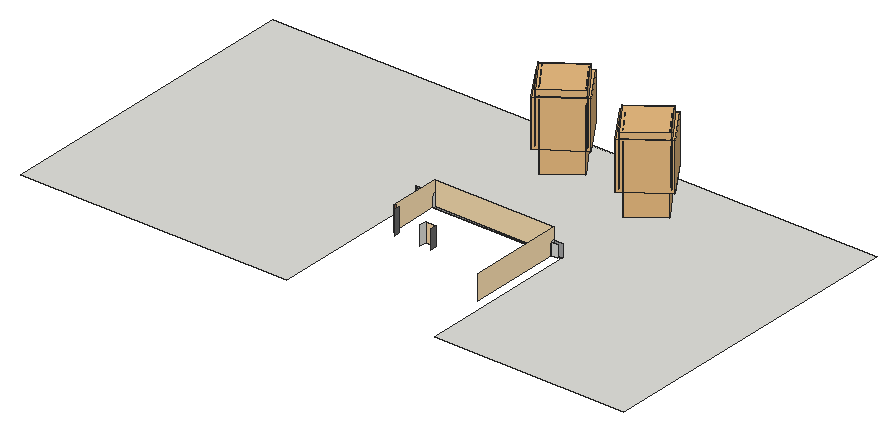
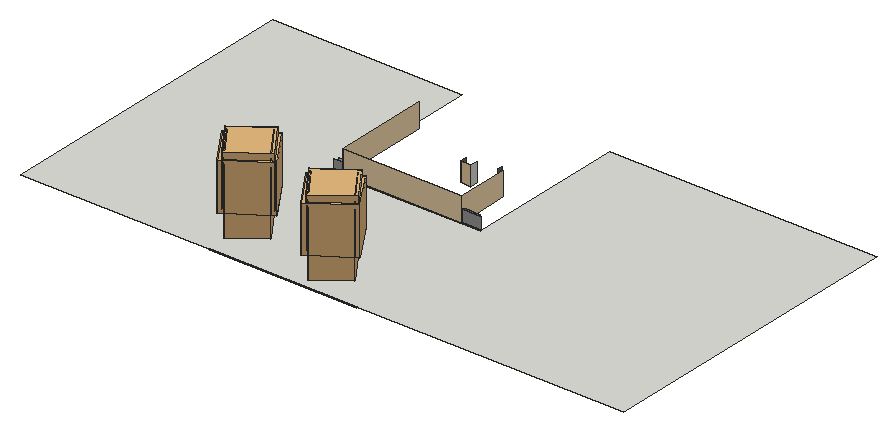
# SketchUp Ruby script. Lengths in inches.
U = 1.inch
M = Sketchup.active_model
def pt(a) = Geom::Point3d.new(a.map { |v| v * U })
def face(e, loops, mat)
  f = e.add_face(loops[0].map { |a| pt(a) })
  loops[1..].each { |l| e.add_face(l.map { |a| pt(a) }).erase! }
  f.material = f.back_material = mat if mat
  f
end
# faces: each face lists its corners as indices into pts; further lists are holes
def faces(e, pts, list, mat = nil) = list.each { |f| face(e, (f[0].is_a?(Array) ? f : [f]).map { |l| l.map { |i| pts[i] } }, mat) }
# xy, xz, yz: faces in a plane at the given z, y or x. An outline is a flat list of corners, or four numbers for a rectangle; further outlines are holes
def ring(l) = l.size == 4 ? [[l[0], l[1]], [l[2], l[1]], [l[2], l[3]], [l[0], l[3]]] : l.each_slice(2).to_a
def flat(e, list, mat, &to3) = list.each { |f| face(e, (f[0].is_a?(Array) ? f : [f]).map { |l| ring(l).map { |u, v| to3.(u, v) } }, mat) }
def xy(e, z, list, mat = nil) = flat(e, list, mat) { |x, y| [x, y, z] }
def xz(e, y, list, mat = nil) = flat(e, list, mat) { |x, z| [x, y, z] }
def yz(e, x, list, mat = nil) = flat(e, list, mat) { |y, z| [x, y, z] }
def lines(e, pts, list) = list.each { |a, b| e.add_line(pt(pts[a]), pt(pts[b])) }
# prism: a flat outline (further loops are holes) pulled along v
def prism(e, loops, v, mat = nil)
  f = face(e, loops, mat); d = Geom::Vector3d.new(v.map { |x| x * U })
  f.pushpull(f.normal.samedirection?(d) ? d.length : -d.length)
end
def box(e, o, s, mat = nil) = prism(e, [[o, [o[0] + s[0], o[1], o[2]], [o[0] + s[0], o[1] + s[1], o[2]], [o[0], o[1] + s[1], o[2]]]], [0, 0, s[2]], mat)
def at(x, y, z, deg = 0) = Geom::Transformation.translation(pt([x, y, z])) * Geom::Transformation.rotation(ORIGIN, Z_AXIS, deg.degrees)
def axes(o, x, y, z) = Geom::Transformation.new([*x, 0, *y, 0, *z, 0, *pt(o).to_a, 1])
def part(name) = M.definitions.add(name)
# library, detail: a bought-in or finely detailed component or shape, given as its bounding box
def library(name, o, s) = part(name).tap { |d| box(d.entities, o, s) }
def detail(e, o, s) = box(e.add_group.entities, o, s)
def put(e, d, t, mat = nil) = e.add_instance(d, t).tap { |i| i.material = mat if mat }
def group(e, t, mat = nil) = e.add_group.tap { |g| g.transformation = t; g.material = mat if mat }.entities
root = M.entities
M.materials.add("028_190k_fullGeometry_Material \#4").color = [120, 148, 64]
M.materials.add("[0032_Moccasin]").color = [255, 228, 181]
M.materials.add("[0033_NavajoWhite]").color = [255, 222, 173]
M.materials.add("[0132_LightGray]").color = [169, 169, 169]
M.materials.add("[0134_DimGray]").color = [105, 105, 105]
M.materials.add("[Tile Ceramic Multi]").color = [165, 115, 84]
c1 = library("028_190k_fullGeometry_0",[-319.99,-281.1,-2.15],[577.33,562.38,1159.36])
c2 = library("028_190k_fullGeometry_1",[-333.4,-281.7,421.48],[600.33,578.53,738.83])
c3 = library("028_190k_fullGeometry_2",[-3584003,-3264710,4041818.25],[6566285.5,6460741.75,7903602.75])
c4 = library("028_190k_fullGeometry_3",[-353.86,-324.57,405.22],[652.24,636.69,781.83])
c5 = part("028_190k_fullGeometry_4")
p = [[125.51,152.8,882.93],[125.36,152.82,883.01],[124.8,155.5625,881.05]]
faces(c5.entities,p,[[0,1,2]],"028_190k_fullGeometry_Material \#4")
c6 = part("028_190k_fullGeometry")
g1 = group(c6.entities,at(0,0,0))
put(g1,c1,axes([0,0,0],[0.18998,-0.26642,0],[0.26642,0.18998,0],[0,0,0.32722]))
put(g1,c2,axes([0,0,0],[0.18998,-0.26642,0],[0.26642,0.18998,0],[0,0,0.32722]))
put(g1,c3,axes([0,0,0],[0.00002,-0.00003,0],[0.00003,0.00002,0],[0,0,0.00003]))
put(g1,c4,axes([0,0,0],[0.18998,-0.26642,0],[0.26642,0.18998,0],[0,0,0.32722]))
put(g1,c5,axes([0,0,0],[0.18998,-0.26642,0],[0.26642,0.18998,0],[0,0,0.32722]))
xy(root,-9,[[1338.625,807.5,2076.625,1583.3125]])
xy(root,-6,[[0,0,1338.625,0,1338.625,807.5,2076.625,807.5,2076.625,0,3026.5,0,3026.5,1583.3125,0,1583.3125]])
xz(root,549.6875,[[1431.3125,0,1437.22,8],[1431.3125,8,1437.22,16],[1431.3125,16,1437.22,24],[1431.3125,24,1437.22,32]],"[Tile Ceramic Multi]")
xz(root,555,[[1437.22,0,1454.9375,8],[1437.22,8,1454.9375,16],[1437.22,16,1454.9375,24],[1437.22,24,1454.9375,32]],"[Tile Ceramic Multi]")
xz(root,560.625,[[1583.17,0,1636.42,95.25]],"[0033_NavajoWhite]")
xz(root,786.1875,[[2031.3125,0,2065.5625,60]])
xz(root,799.5,[[1346.625,0,1431.3125,60]],"[0132_LightGray]")
xz(root,807.5,[[1431.3125,0,2031.3125,120]],"[0032_Moccasin]")
xz(root,807.5,[[1338.625,-6,1338.625,0,2031.3125,0,2031.3125,60,2076.625,60,2076.625,-6],[1338.625,0,1431.3125,60]],"[0132_LightGray]")
xz(root,1583.3125,[[1338.625,-9,2076.625,-6]])
yz(root,1431.3125,[[799.5,0,807.5,60]])
yz(root,1431.3125,[[549.6875,0,549.6875,120,807.5,120,807.5,60,799.5,60,799.5,0]],"[0032_Moccasin]")
yz(root,1437.22,[[549.6875,0,555,120]],"[Tile Ceramic Multi]")
yz(root,1454.9375,[[528.0625,0,555,120]],"[0134_DimGray]")
yz(root,1583.17,[[528.0625,0,560.625,95.25]])
yz(root,1636.42,[[528.0625,0,560.625,95.25]],"[0134_DimGray]")
yz(root,2031.3125,[[786.1875,0,807.5,60]])
yz(root,2031.3125,[[327.5,0,786.1875,0,786.1875,60,807.5,60,807.5,120,327.5,120]],"[0032_Moccasin]")
put(root,c6,at(2075.72,1336.63,-5.3))
put(root,c6,at(1607.5625,1396.26,-5.3))
